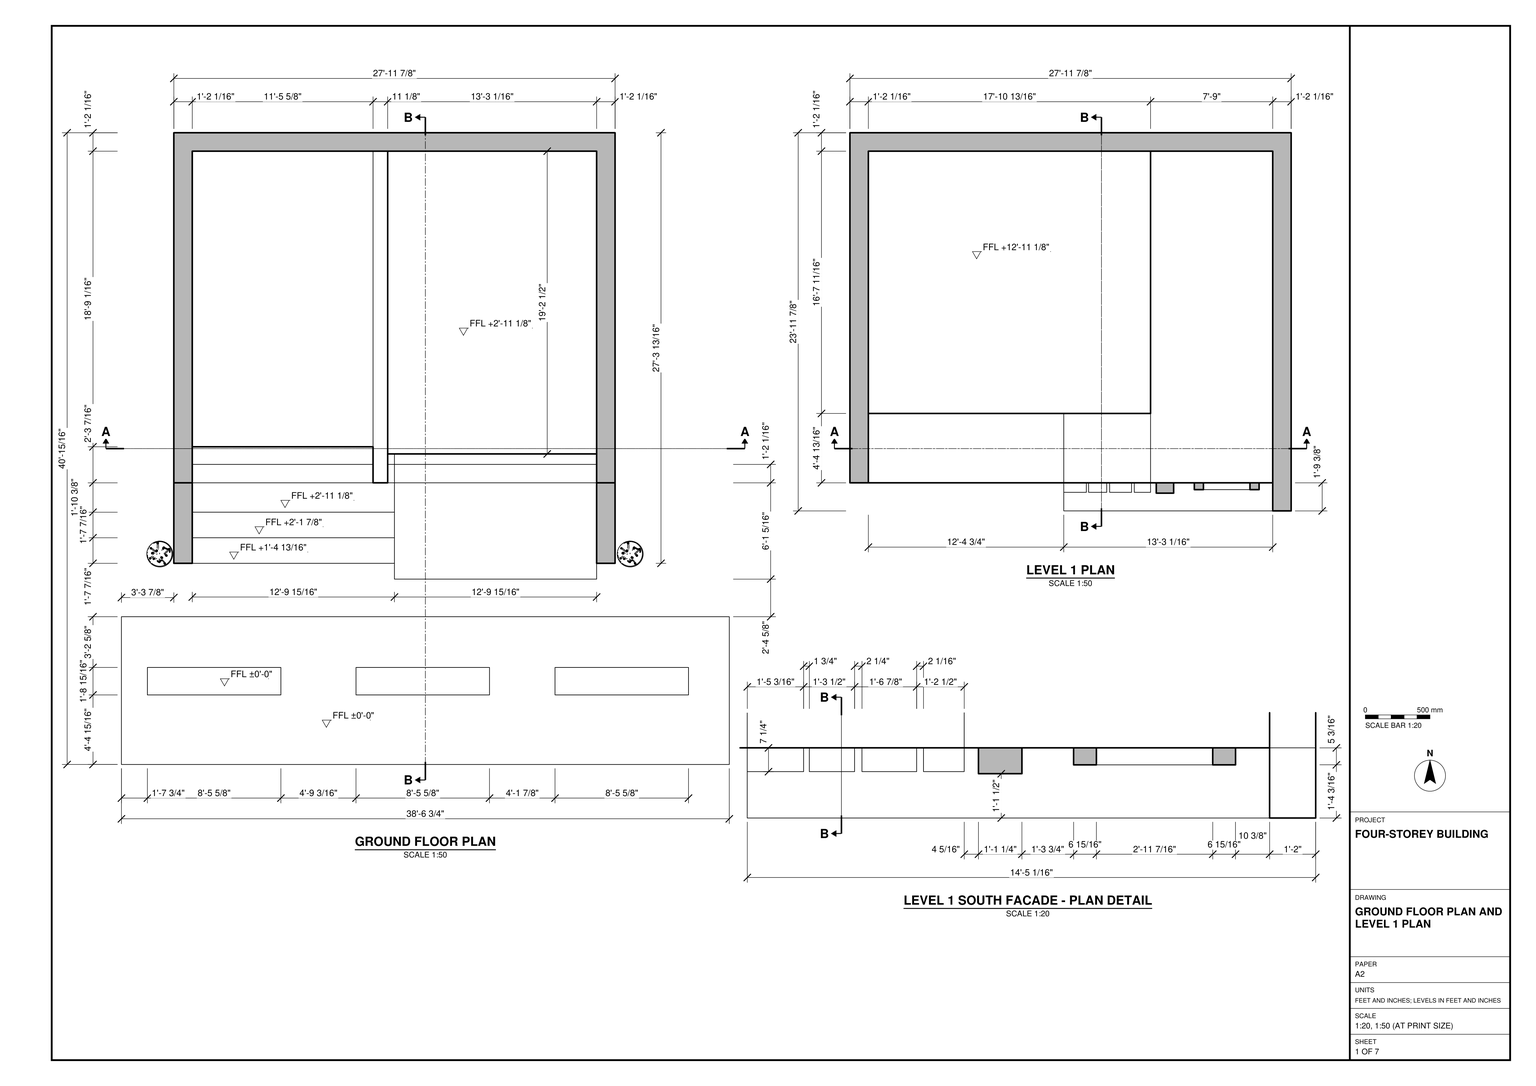
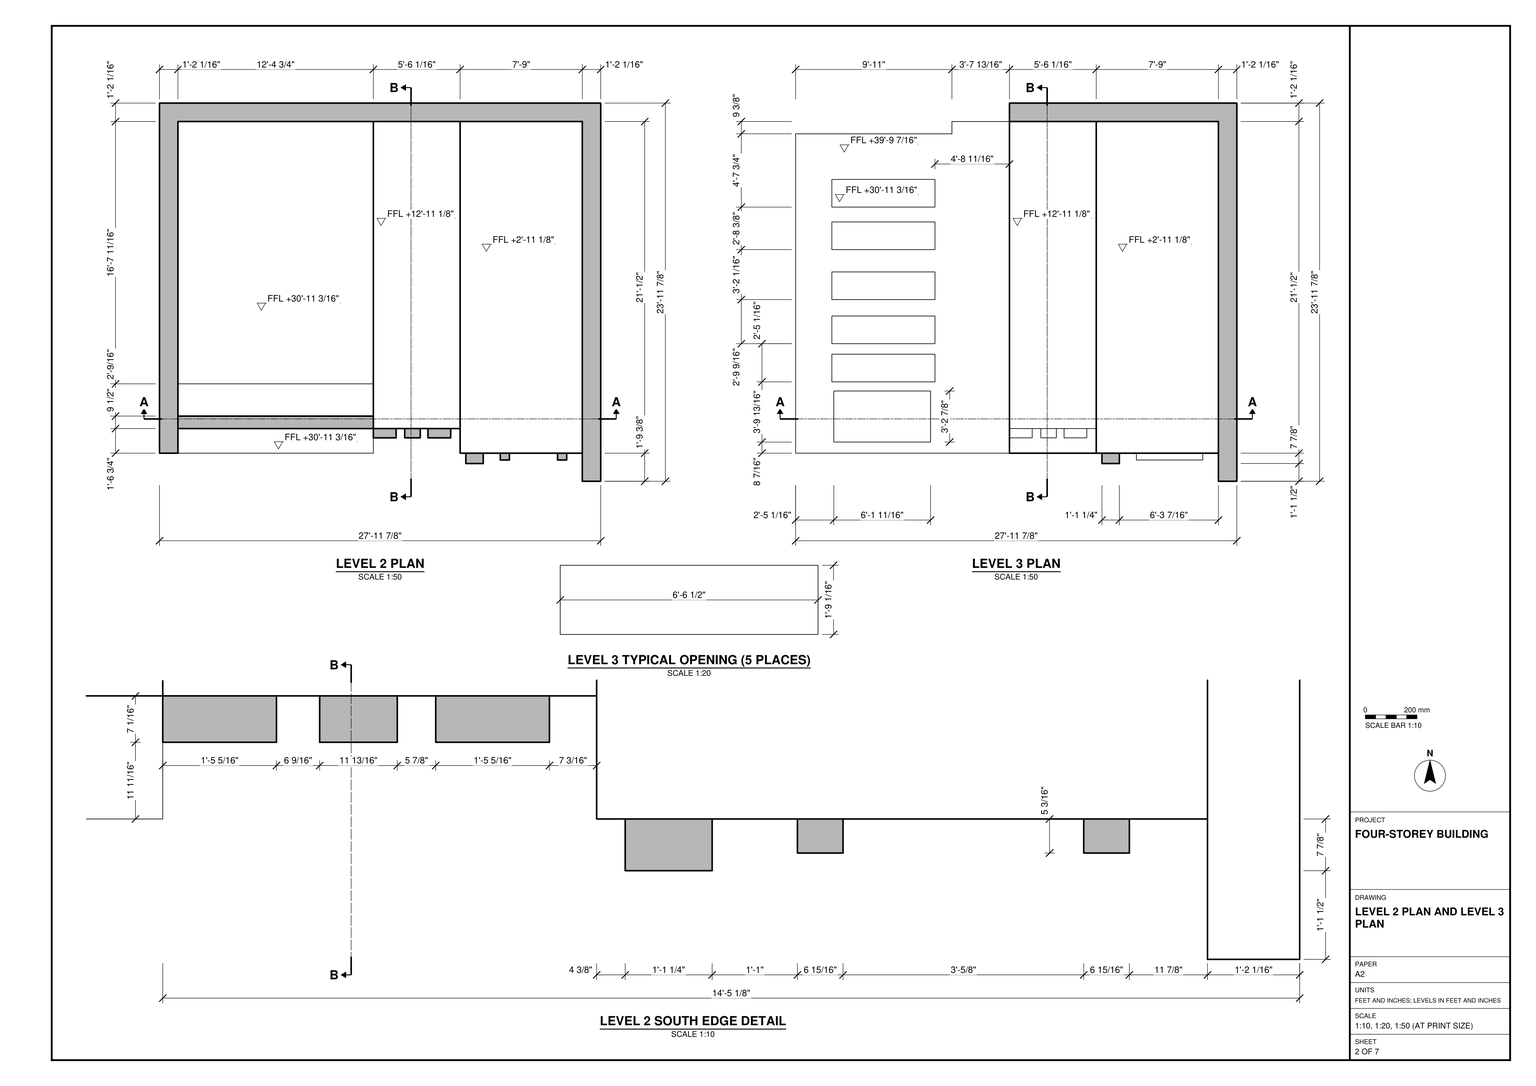
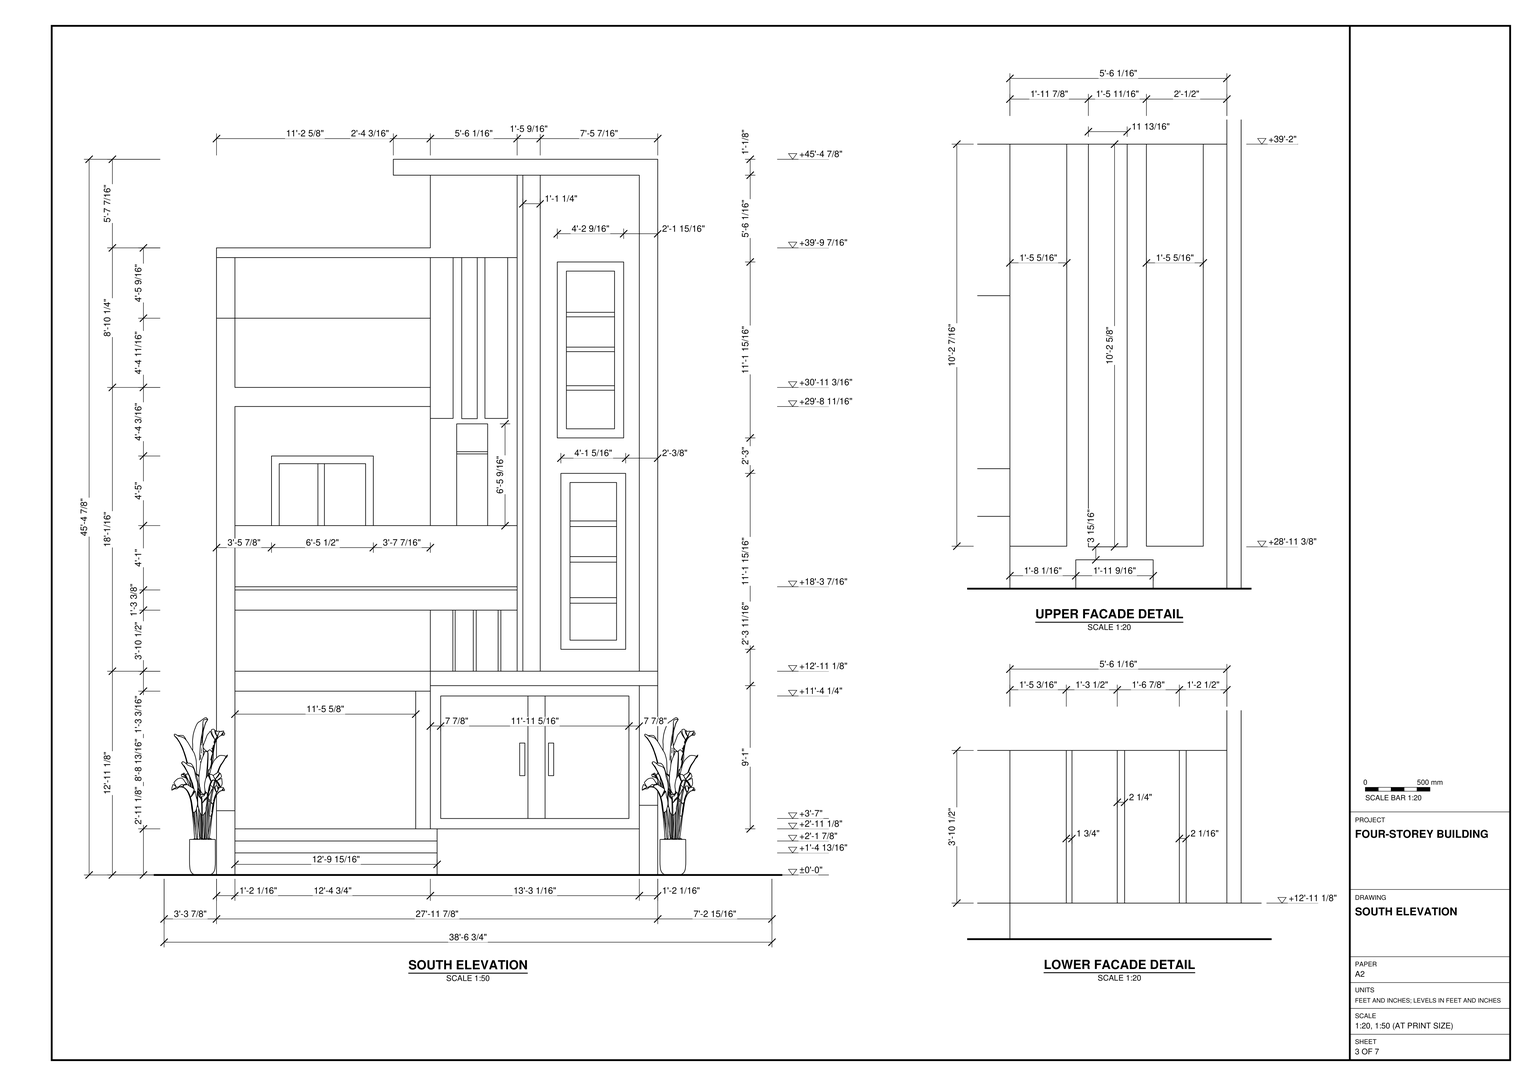
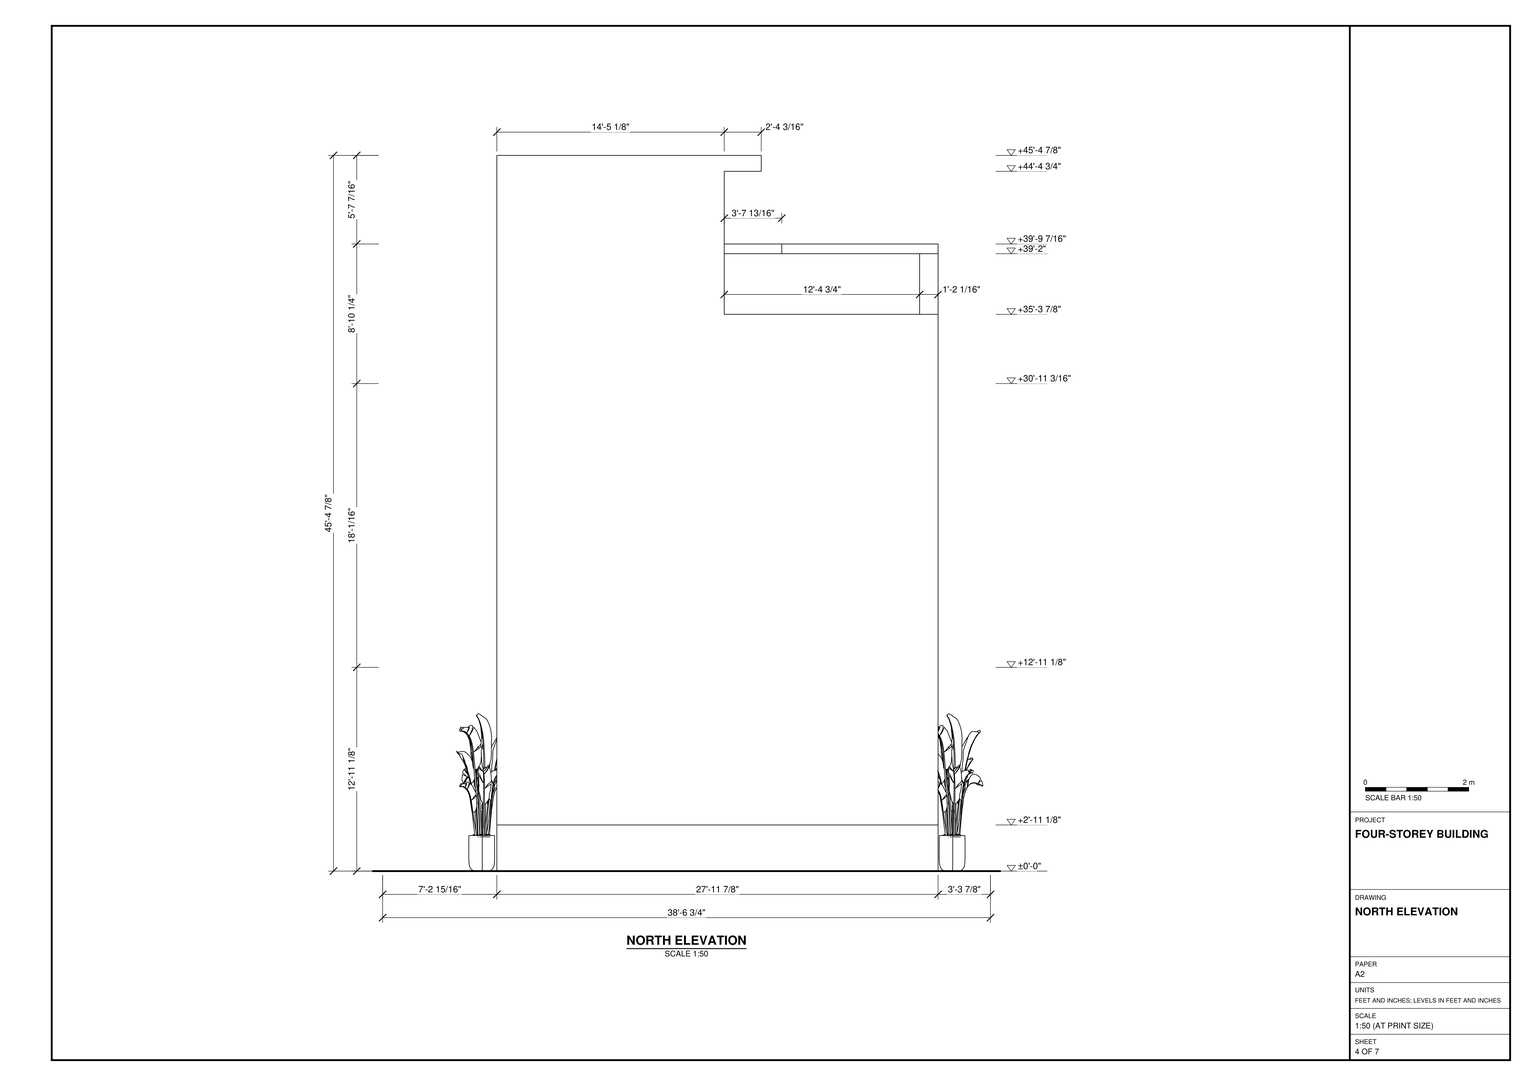
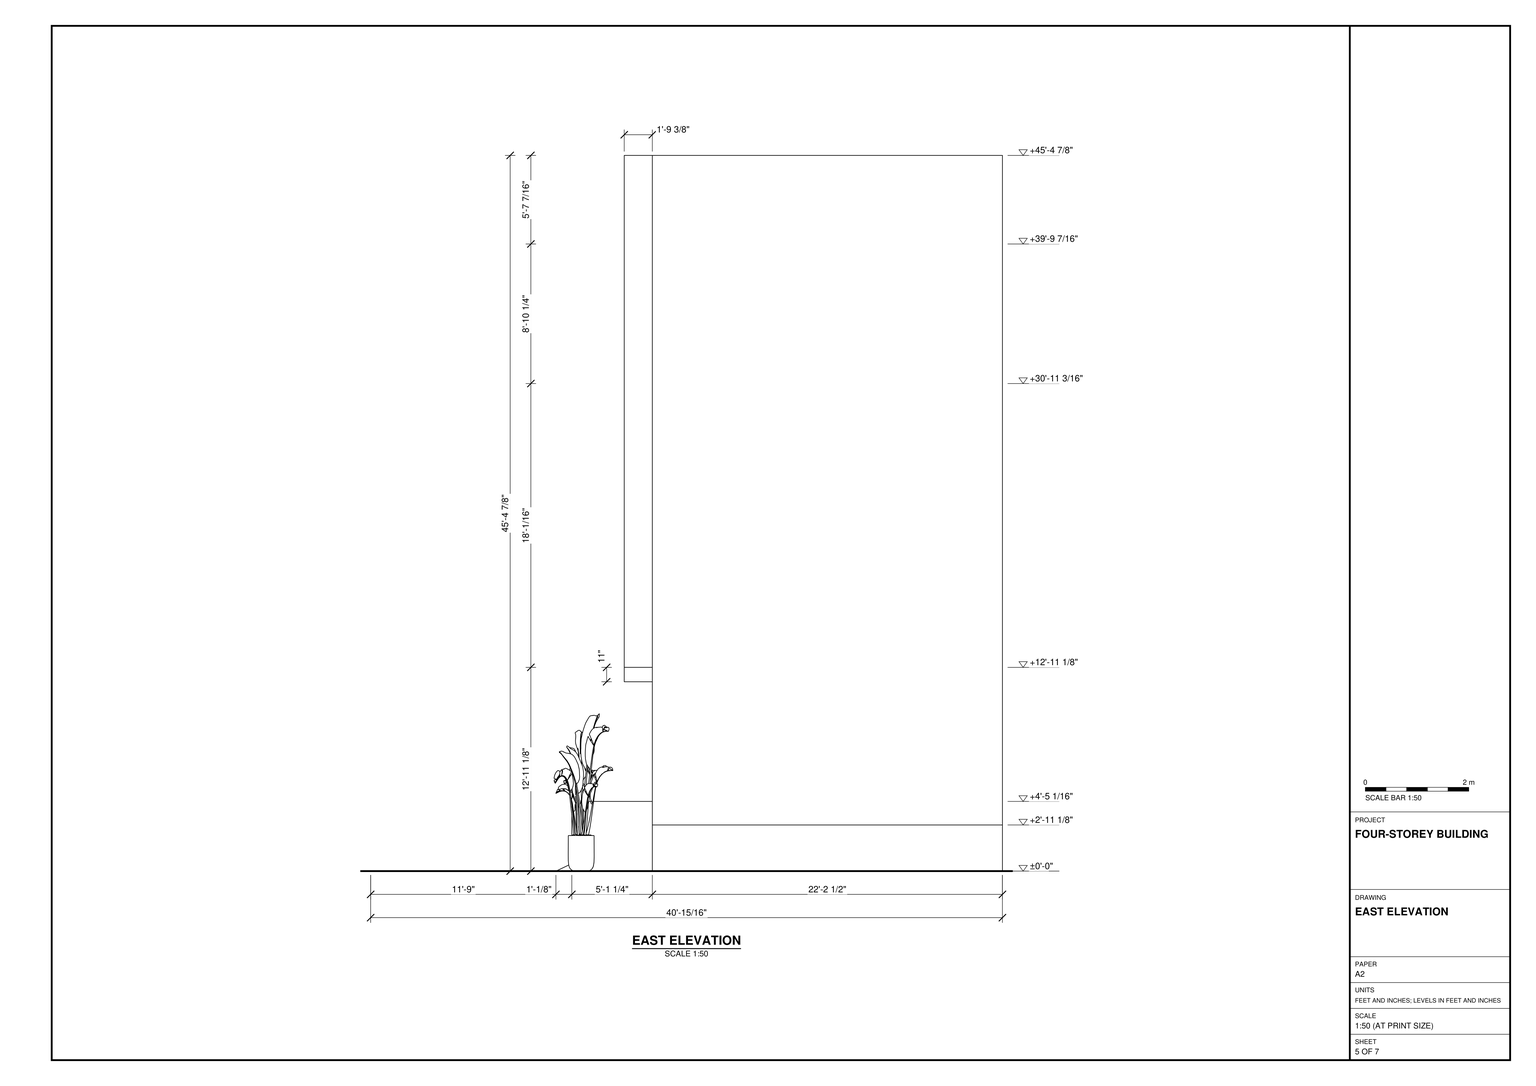
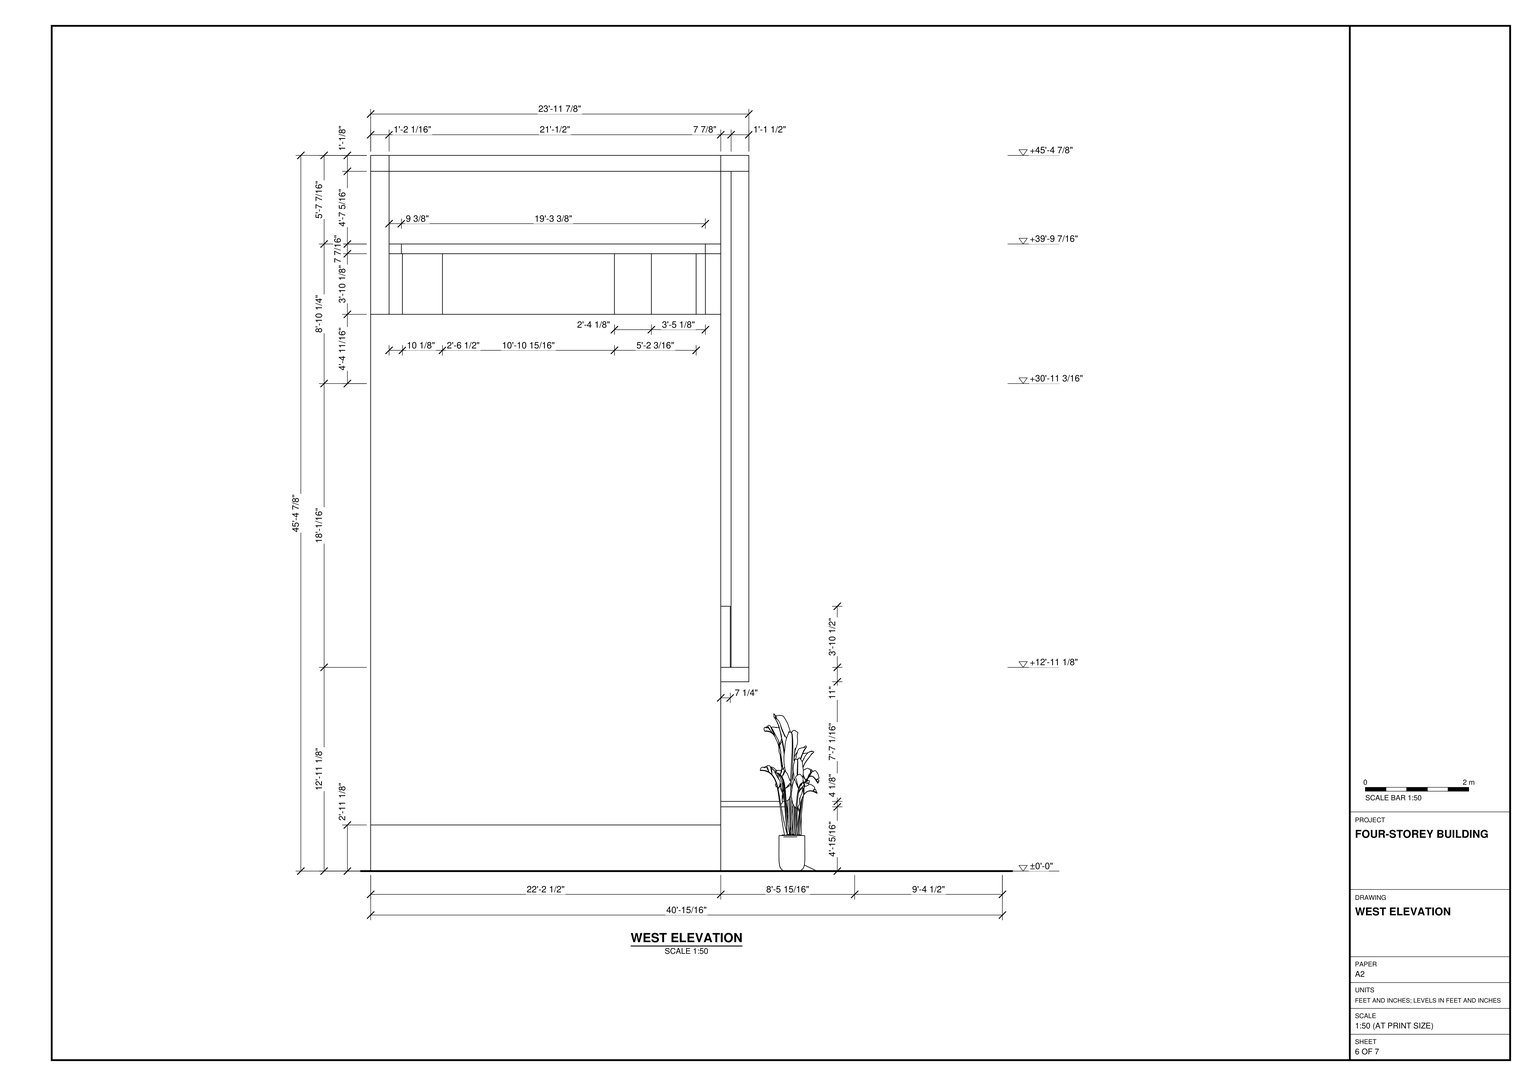
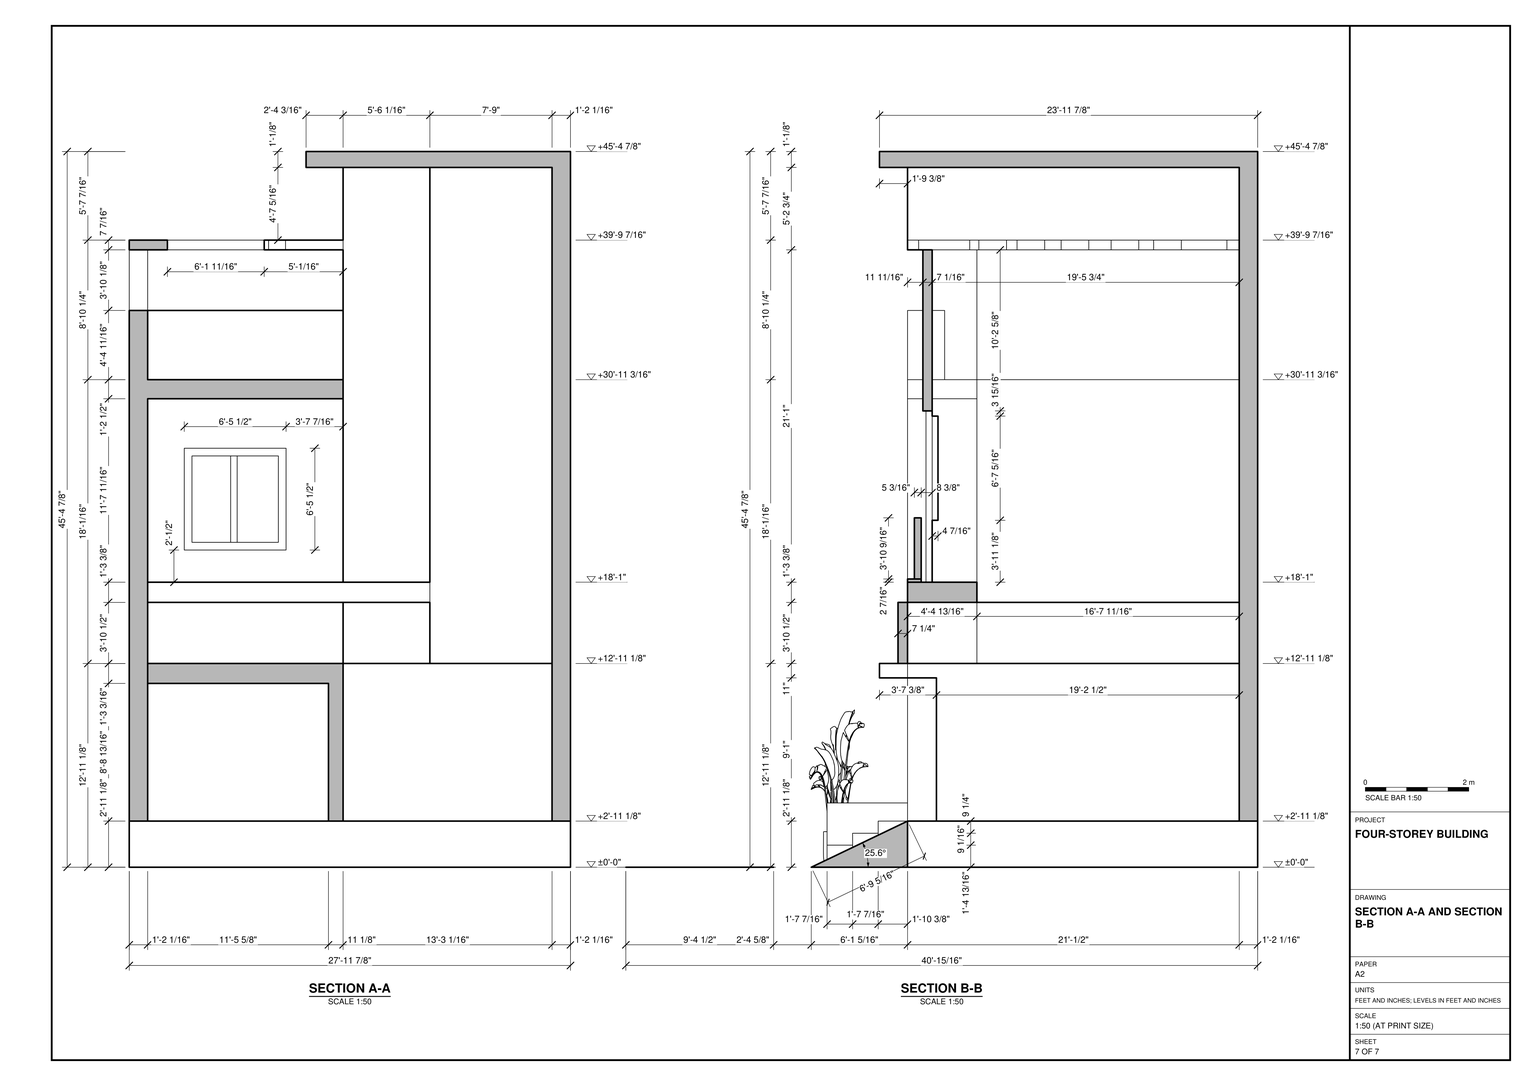
Build the four-storey building in SketchUp using task_files/diagram_01.pdf. Work in feet and inches, with X running east–west and Y running north–south. Including the forecourt and roof, the overall extents are 38'-6 3/4" along X, 40'-15/16" along Y and 45'-4 7/8" in height. Set the ground datum at ±0'-0", Level 1 at +12'-11 1/8", Level 2 at +30'-11 3/16" and Level 3 at +39'-9 7/16".

Distinguish the wider forecourt from the 27'-11 7/8" building body. Model the rear and side walls at their drawn thickness of 1'-2 1/16", the ground-floor dividing wall, the raised floor and the broad steps in the west entrance bay. Place the paired entrance doors in the east bay. Follow the slab outline at each level, retaining the areas open to the floors below. Cut the row of rectangular openings in the western Level 3 slab.

Use the south elevation and edge details to position the horizontal bands, narrow vertical projections, stacked window units and projecting flat roof. Include the planters flanking the entrance. Decor and loose items, including plants, may be suitable library components. Keep walls, slabs, roof and each furniture or joinery piece shown in separate groups or components, and use components for repeated parts. Save one SketchUp model as output_files/four_storey_building_with_its_stepped_south_facade.skp.

# SketchUp Ruby script. Lengths in inches.
U = 1.inch
M = Sketchup.active_model
def pt(a) = Geom::Point3d.new(a.map { |v| v * U })
def face(e, loops, mat)
  f = e.add_face(loops[0].map { |a| pt(a) })
  loops[1..].each { |l| e.add_face(l.map { |a| pt(a) }).erase! }
  f.material = f.back_material = mat if mat
  f
end
# faces: each face lists its corners as indices into pts; further lists are holes
def faces(e, pts, list, mat = nil) = list.each { |f| face(e, (f[0].is_a?(Array) ? f : [f]).map { |l| l.map { |i| pts[i] } }, mat) }
# xy, xz, yz: faces in a plane at the given z, y or x. An outline is a flat list of corners, or four numbers for a rectangle; further outlines are holes
def ring(l) = l.size == 4 ? [[l[0], l[1]], [l[2], l[1]], [l[2], l[3]], [l[0], l[3]]] : l.each_slice(2).to_a
def flat(e, list, mat, &to3) = list.each { |f| face(e, (f[0].is_a?(Array) ? f : [f]).map { |l| ring(l).map { |u, v| to3.(u, v) } }, mat) }
def xy(e, z, list, mat = nil) = flat(e, list, mat) { |x, y| [x, y, z] }
def xz(e, y, list, mat = nil) = flat(e, list, mat) { |x, z| [x, y, z] }
def yz(e, x, list, mat = nil) = flat(e, list, mat) { |y, z| [x, y, z] }
def lines(e, pts, list) = list.each { |a, b| e.add_line(pt(pts[a]), pt(pts[b])) }
# prism: a flat outline (further loops are holes) pulled along v
def prism(e, loops, v, mat = nil)
  f = face(e, loops, mat); d = Geom::Vector3d.new(v.map { |x| x * U })
  f.pushpull(f.normal.samedirection?(d) ? d.length : -d.length)
end
def box(e, o, s, mat = nil) = prism(e, [[o, [o[0] + s[0], o[1], o[2]], [o[0] + s[0], o[1] + s[1], o[2]], [o[0], o[1] + s[1], o[2]]]], [0, 0, s[2]], mat)
def at(x, y, z, deg = 0) = Geom::Transformation.translation(pt([x, y, z])) * Geom::Transformation.rotation(ORIGIN, Z_AXIS, deg.degrees)
def axes(o, x, y, z) = Geom::Transformation.new([*x, 0, *y, 0, *z, 0, *pt(o).to_a, 1])
def part(name) = M.definitions.add(name)
# library, detail: a bought-in or finely detailed component or shape, given as its bounding box
def library(name, o, s) = part(name).tap { |d| box(d.entities, o, s) }
def detail(e, o, s) = box(e.add_group.entities, o, s)
def put(e, d, t, mat = nil) = e.add_instance(d, t).tap { |i| i.material = mat if mat }
def group(e, t, mat = nil) = e.add_group.tap { |g| g.transformation = t; g.material = mat if mat }.entities
root = M.entities
M.materials.add("[Asphalt New]").color = [67, 60, 62]
M.materials.add("[Blinds Roman Hobbled Blue]").color = [49, 50, 53]
M.materials.add("[Blinds Vertical Pattern]").color = [232, 232, 234]
M.materials.add("[Blinds Vertical Pattern]1").color = [247, 247, 249]
M.materials.add("[Color C08]").color = [79, 39, 0]
M.materials.add("[Color C08]1").color = [102, 51, 0]
M.materials.add("[Color M00]").color = [255, 255, 255]
M.materials.add("[Color M06]").color = [86, 86, 86]
M.materials.add("[Formica Beige]").color = [211, 187, 149]
M.materials.add("[Formica Laminate Dark]").color = [50, 53, 60]
M.materials.add("[Formica Laminate Light]").color = [213, 189, 164]
M.materials.add("[Formica Speckled Grey]").color = [94, 105, 111]
M.materials.add("[Sandstone]").color = [118, 81, 52]
M.materials.add("[Terrazzo Tile Light]").color = [219, 217, 210]
M.materials.add("[Translucent Glass Gray]").color = [128, 128, 128]
M.materials["[Translucent Glass Gray]"].alpha = 0.5
M.materials.add("[Translucent Glass Safety]").color = [213, 245, 255]
M.materials["[Translucent Glass Safety]"].alpha = 0.19
M.materials.add("[Translucent Glass Safety]1").color = [204, 235, 244]
M.materials["[Translucent Glass Safety]1"].alpha = 0.5
M.materials.add("[Wood Cherry Original]").color = [152, 86, 42]
M.materials.add("[Wood Floor Light]").color = [204, 176, 127]
M.materials.add("[Wood Floor Parquet]").color = [145, 89, 39]
M.materials.add("[Wood Floor]").color = [155, 105, 61]
M.materials.add("[Wood Veneer 01]").color = [63, 37, 19]
M.materials.add("[Wood Veneer 01]1").color = [120, 70, 37]
M.materials.add("[Wood Veneer 02]").color = [190, 128, 91]
c1 = library("chau cay",[-24.34,-109.24,0],[56.46,62.58,79.69])
xy(root,0,[[207.84,141.12,361.75,153.16],[39.89,153.16,39.89,480.95,375.78,480.95,375.78,214.43,53.92,214.43,53.92,153.16],[53.92,153.16,207.84,172.61],[207.84,153.16,361.75,214.43],[361.75,153.16,375.78,214.43],
  [53.92,172.61,207.84,192.07],[53.92,192.07,207.84,214.43]])
xy(root,0,[[19.76,52.95,121.39,73.89],[178.57,52.95,280.2,73.89],[330.07,52.95,431.7,73.89]],"[Color M00]")
xy(root,0,[[[0,0,462.75,112.5],[19.76,52.95,121.39,73.89],[178.57,52.95,280.2,73.89],[330.07,52.95,431.7,73.89]]],"[Color M06]")
xy(root,16.8125,[[53.92,153.16,207.84,172.61]],"[Terrazzo Tile Light]")
xy(root,25.875,[[53.92,172.61,207.84,192.07]],"[Terrazzo Tile Light]")
xy(root,35.125,[[39.89,214.43,39.89,480.95,375.78,480.95,375.78,214.43,361.75,214.43,361.75,466.92,53.92,466.92,53.92,214.43],[191.55,214.43,202.6875,466.92],[202.6875,236.43,361.75,466.92],[53.92,241.87,191.55,466.92]])
xy(root,35.125,[[53.92,192.07,207.84,214.43],[53.92,214.43,191.55,228.46],[202.6875,214.43,207.84,228.46],[207.84,214.43,361.75,228.46],[53.92,228.46,191.55,241.87],
  [202.6875,228.46,207.84,236.43],[207.84,228.46,361.75,236.43]],"[Terrazzo Tile Light]")
xy(root,48.9375,[[39.89,153.16,53.92,214.43]],"[Terrazzo Tile Light]")
xy(root,53.0625,[[361.75,153.16,375.78,214.43]],"[Terrazzo Tile Light]")
xy(root,139.93,[[53.92,214.43,191.55,241.87]],"[Asphalt New]")
xy(root,144.15,[[202.6875,193.05,202.6875,236.43,361.75,236.43,361.75,214.43,375.78,214.43,375.78,193.05]],"[Blinds Vertical Pattern]")
xy(root,155.125,[[361.75,193.05,375.78,214.43],[273.09,206.55,286.33,214.43],[202.6875,207.18,219.85,214.43],[221.59,207.18,235.375,214.43],[237.62,207.18,254.28,214.43],
  [256.36,207.18,268.75,214.43],[202.6875,214.43,268.75,466.92],[268.75,214.43,361.75,466.92],[53.92,267.23,191.55,466.92],[191.55,267.23,202.6875,466.92]])
xy(root,155.125,[[202.6875,193.05,361.75,193.05,361.75,214.43,286.33,214.43,286.33,206.55,273.09,206.55,273.09,214.43,268.75,214.43,268.75,207.18,256.36,207.18,256.36,214.43,254.28,214.43,254.28,207.18,237.62,207.18,237.62,214.43,235.375,214.43,235.375,207.18,221.59,207.18,221.59,214.43,219.85,214.43,219.85,207.18,202.6875,207.18],[53.92,214.43,191.55,267.23],[191.55,214.43,202.6875,267.23]],"[Blinds Vertical Pattern]")
xy(root,171.81,[[302.07,209.24,351.38,214.43]],"[Color C08]")
xy(root,178.76,[[309.01,209.24,344.43,214.43]],"[Color C08]")
xy(root,201.625,[[202.6875,214.43,268.75,267.23],[53.92,267.23,268.75,466.92]])
xy(root,201.625,[[53.92,214.43,202.6875,267.23]],"[Wood Cherry Original]")
xy(root,201.625,[[202.6875,207.18,219.85,214.43],[221.59,207.18,235.375,214.43],[237.62,207.18,254.28,214.43],[256.36,207.18,268.75,214.43]],"[Wood Veneer 02]")
xy(root,216.99,[[53.92,214.43,268.75,224.81],[53.92,224.81,202.6875,267.23],[202.6875,224.81,268.75,233.17],[202.6875,233.17,268.75,267.23]])
xy(root,219.43,[[53.92,214.43,268.75,219.62],[53.92,219.62,268.75,224.81]])
xy(root,264.13,[[222.75,233.17,246.31,237.61]],"[Formica Laminate Light]")
xy(root,265.99,[[53.92,219.62,268.75,224.81]])
xy(root,298.8,[[309.01,209.24,344.43,214.43]],"[Color C08]")
xy(root,305.75,[[302.07,209.24,351.38,214.43]],"[Wood Veneer 01]1")
xy(root,332.75,[[299.32,209.24,349.86,214.43]],"[Color C08]")
xy(root,339.69,[[306.26,209.24,342.91,214.43]],"[Color C08]")
xy(root,343.44,[[222.75,233.17,246.31,237.61]],"[Formica Laminate Light]")
xy(root,347.39,[[226.58,226.11,238.39,233.17]],"[Wood Veneer 02]")
xy(root,347.58,[[202.6875,226.11,220,233.17],[244.25,226.11,261.5625,233.17]],"[Wood Veneer 02]")
xy(root,356.67,[[53.92,214.43,202.6875,228.46]],"[Blinds Vertical Pattern]")
xy(root,356.67,[[53.92,228.46,202.6875,267.23]],"[Wood Cherry Original]")
xy(root,371.1875,[[53.92,214.43,202.6875,233.17],[53.92,233.17,202.6875,242.66],[53.92,242.66,202.6875,267.23],[53.92,267.23,202.6875,466.92]])
xy(root,423.875,[[39.89,267.23,53.92,295.36],[39.89,426.29,53.92,456.77]])
xy(root,423.875,[[39.89,214.43,53.92,267.23],[53.92,233.17,202.6875,242.66],[39.89,295.36,53.92,426.29],[39.89,456.77,53.92,456.77,53.92,466.92,202.6875,466.92,202.6875,480.95,39.89,480.95]],"[Blinds Vertical Pattern]")
xy(root,459.74,[[306.26,209.24,342.91,214.43]],"[Sandstone]")
xy(root,466.68,[[299.32,209.24,349.86,214.43]],"[Color C08]")
xy(root,470.02,[[202.6875,226.11,220,233.17],[226.58,226.11,238.39,233.17],[244.25,226.11,261.5625,233.17]])
xy(root,470.02,[[[39.89,214.43,39.89,267.23,53.92,267.23,53.92,295.36,39.89,295.36,39.89,426.29,53.92,426.29,53.92,456.77,39.89,456.77,39.89,457.55,158.875,457.55,158.875,466.92,202.6875,466.92,202.6875,226.11,220,226.11,220,233.17,226.58,233.17,226.58,226.11,238.39,226.11,238.39,233.17,244.25,233.17,244.25,226.11,261.5625,226.11,261.5625,233.17,268.75,233.17,268.75,214.43],[164.65,234.83,193.97,419.64],[68.95,222.9,142.63,261.77],[67.48,297.78,145.98,318.84],[67.48,331.34,145.98,352.41],[67.48,268.72,145.98,289.78],[67.48,369.41,145.98,390.47],[67.48,401.78,145.98,422.84]]],"[Blinds Vertical Pattern]")
xy(root,470.02,[[168.46,238.63,190.16,415.84]],"[Color C08]1")
xy(root,470.02,[[[164.65,234.83,193.97,419.64],[168.46,238.63,190.16,415.84]]],"[Formica Beige]")
xy(root,477.4375,[[[39.89,214.43,202.6875,214.43,202.6875,466.92,158.875,466.92,158.875,457.55,39.89,457.55],[68.95,222.9,142.63,261.77],[67.48,331.34,145.98,352.41],[67.48,297.78,145.98,318.84],[67.48,369.41,145.98,390.47],[67.48,268.72,145.98,289.78],[67.48,401.78,145.98,422.84]]],"[Blinds Vertical Pattern]")
xy(root,532.75,[[273.09,206.55,286.33,214.43],[202.6875,214.43,268.75,228.46],[268.75,214.43,361.75,228.46],[202.6875,228.46,268.75,466.92],[268.75,228.46,361.75,466.92],
  [174.5,466.92,202.6875,480.95]])
xy(root,532.75,[[174.5,193.05,174.5,466.92,202.6875,466.92,202.6875,214.43,273.09,214.43,273.09,206.55,286.33,206.55,286.33,214.43,361.75,214.43,361.75,193.05]],"[Blinds Vertical Pattern]")
xy(root,544.875,[[174.5,193.05,375.78,214.43],[174.5,214.43,375.78,480.95]],"[Blinds Vertical Pattern]1")
xz(root,153.16,[[39.89,0,53.92,48.9375],[53.92,0,207.84,16.8125],[361.75,0,375.78,53.0625]],"[Terrazzo Tile Light]")
xz(root,172.61,[[53.92,0,207.84,16.8125]])
xz(root,172.61,[[53.92,16.8125,207.84,25.875]],"[Terrazzo Tile Light]")
xz(root,192.07,[[53.92,0,207.84,25.875]])
xz(root,192.07,[[53.92,25.875,207.84,35.125]],"[Terrazzo Tile Light]")
xz(root,193.05,[[202.6875,144.15,375.78,155.125],[361.75,155.125,375.78,155.125,375.78,544.875,174.5,544.875,174.5,532.75,361.75,532.75]],"[Blinds Vertical Pattern]")
xz(root,206.55,[[273.09,155.125,286.33,532.75]],"[Wood Veneer 02]")
xz(root,207.18,[[202.6875,155.125,219.85,201.625],[221.59,155.125,235.375,201.625],[237.62,155.125,254.28,201.625],[256.36,155.125,268.75,201.625]],"[Wood Veneer 02]")
xz(root,209.24,[[[302.07,171.81,351.38,305.75],[309.01,178.76,344.43,298.8]],[[299.32,332.75,349.86,466.68],[306.26,339.69,342.91,459.74]]],"[Color C08]")
xz(root,214.43,[[53.92,0,207.84,35.125],[207.84,0,361.75,35.125],[361.75,0,375.78,35.125],[39.89,35.125,53.92,48.9375],[361.75,35.125,375.78,53.0625],
  [361.75,144.15,375.78,155.125],[202.6875,155.125,219.85,201.625],[219.85,155.125,221.59,201.625],[221.59,155.125,235.375,201.625],[235.375,155.125,237.62,201.625],
  [237.62,155.125,254.28,201.625],[254.28,155.125,256.36,201.625],[256.36,155.125,268.75,201.625],[273.09,155.125,286.33,532.75],[[302.07,171.81,351.38,305.75],[309.01,178.76,344.43,298.8]],
  [53.92,216.99,268.75,219.43],[[299.32,332.75,349.86,466.68],[306.26,339.69,342.91,459.74]]])
xz(root,214.43,[[53.92,139.93,202.6875,155.125]],"[Asphalt New]")
xz(root,214.43,[[191.55,35.125,202.6875,139.93],[361.75,53.0625,375.78,144.15],[268.75,155.125,273.09,532.75],[[286.33,155.125,361.75,532.75],[299.32,332.75,349.86,466.68],[302.07,171.81,351.38,305.75]],[39.89,470.02,268.75,470.02,268.75,532.75,202.6875,532.75,202.6875,477.4375,39.89,477.4375]],"[Blinds Vertical Pattern]")
xz(root,214.43,[[39.89,48.9375,53.92,48.9375,53.92,356.67,202.6875,356.67,202.6875,371.1875,53.92,371.1875,53.92,423.875,39.89,423.875],[53.92,201.625,268.75,216.99]],"[Blinds Vertical Pattern]1")
xz(root,214.43,[[309.01,178.76,344.43,206.89],[309.01,206.89,344.43,211.14],[309.01,211.14,344.43,238.14],[309.01,238.14,344.43,242.39],[309.01,242.39,344.43,265.27],
  [309.01,265.27,344.43,269.52],[309.01,269.52,344.43,298.8],[306.26,339.69,342.91,369.05],[306.26,369.05,342.91,372.5],[306.26,372.5,342.91,398.42],
  [306.26,398.42,342.91,401.86],[306.26,401.86,342.91,424.92],[306.26,424.92,342.91,428.36],[306.26,428.36,342.91,459.74]],"[Sandstone]")
xz(root,219.62,[[53.92,219.43,268.75,265.99]],"[Translucent Glass Safety]")
xz(root,222.9,[[68.95,470.02,142.63,477.4375]],"[Blinds Vertical Pattern]")
xz(root,224.81,[[53.92,216.99,202.6875,219.43],[202.6875,216.99,268.75,219.43]])
xz(root,224.81,[[53.92,219.43,202.6875,265.99],[202.6875,219.43,268.75,265.99]],"[Translucent Glass Safety]")
xz(root,226.11,[[226.58,347.39,238.39,470.02],[202.6875,347.58,220,470.02],[244.25,347.58,261.5625,470.02]],"[Wood Veneer 02]")
xz(root,233.17,[[226.58,347.39,238.39,470.02],[202.6875,347.58,220,470.02],[244.25,347.58,261.5625,470.02]])
xz(root,233.17,[[[202.6875,216.99,204.91,216.99,204.91,262.18,217.35,262.18,217.35,216.99,221.29,216.99,221.29,262.18,233.72,262.18,233.72,216.99,238.1,216.99,238.1,262.18,250.54,262.18,250.54,216.99,256.3125,216.99,256.3125,262.18,268.75,262.18,268.75,470.02,261.5625,470.02,261.5625,347.58,244.25,347.58,244.25,470.02,238.39,470.02,238.39,347.39,226.58,347.39,226.58,470.02,220,470.02,220,347.58,202.6875,347.58],[222.75,264.13,246.31,343.44]]],"[Blinds Vertical Pattern]1")
xz(root,233.17,[[53.92,371.1875,202.6875,423.875]],"[Translucent Glass Safety]1")
xz(root,233.17,[[204.91,216.99,217.35,262.18],[221.29,216.99,233.72,262.18],[238.1,216.99,250.54,262.18],[256.3125,216.99,268.75,262.18]],"[Wood Floor Parquet]")
xz(root,236.43,[[[202.6875,35.125,361.75,144.15],[210.57,43.01,353.87,136.27]]],"[Blinds Vertical Pattern]")
xz(root,236.43,[[270.67,75.625,274.65,100.44],[292.61,75.625,296.59,100.44]],"[Formica Laminate Dark]")
xz(root,236.43,[[[210.57,43.01,277,136.27],[270.67,75.625,274.65,100.44]],[277,43.01,290.04,136.27],[[290.04,43.01,353.87,136.27],[292.61,75.625,296.59,100.44]]],"[Wood Veneer 01]")
xz(root,237.61,[[222.75,320.57,246.31,322.24]],"[Formica Speckled Grey]")
xz(root,237.61,[[222.75,322.24,246.31,343.44]],"[Wood Floor Light]")
xz(root,237.61,[[222.75,264.13,246.31,320.57]],"[Wood Floor]")
xz(root,241.87,[[53.92,35.125,191.55,139.93]],"[Blinds Roman Hobbled Blue]")
xz(root,242.66,[[53.92,371.1875,202.6875,423.875]],"[Translucent Glass Safety]1")
xz(root,261.77,[[68.95,470.02,142.63,477.4375]],"[Blinds Vertical Pattern]")
xz(root,267.23,[[53.92,201.625,268.75,216.99],[53.92,356.67,202.6875,371.1875]])
xz(root,267.23,[[53.92,155.125,202.6875,201.625],[[53.92,216.99,202.6875,356.67],[81.78,241.48,159.28,318.98]],[39.89,423.875,53.92,470.02]],"[Blinds Vertical Pattern]")
xz(root,267.23,[[[81.78,241.48,159.28,318.98],[87.64,247.35,153.41,313.12]],[117.09,247.35,122.04,313.12]],"[Formica Laminate Dark]")
xz(root,267.23,[[87.64,247.35,117.09,313.12],[122.04,247.35,153.41,313.12]],"[Translucent Glass Gray]")
xz(root,268.72,[[67.48,470.02,145.98,477.4375]],"[Blinds Vertical Pattern]")
xz(root,289.78,[[67.48,470.02,145.98,477.4375]],"[Blinds Vertical Pattern]")
xz(root,295.36,[[39.89,423.875,53.92,470.02]],"[Blinds Vertical Pattern]")
xz(root,297.78,[[67.48,470.02,145.98,477.4375]],"[Blinds Vertical Pattern]")
xz(root,318.84,[[67.48,470.02,145.98,477.4375]],"[Blinds Vertical Pattern]")
xz(root,331.34,[[67.48,470.02,145.98,477.4375]],"[Blinds Vertical Pattern]")
xz(root,352.41,[[67.48,470.02,145.98,477.4375]],"[Blinds Vertical Pattern]")
xz(root,369.41,[[67.48,470.02,145.98,477.4375]],"[Blinds Vertical Pattern]")
xz(root,390.47,[[67.48,470.02,145.98,477.4375]],"[Blinds Vertical Pattern]")
xz(root,401.78,[[67.48,470.02,145.98,477.4375]],"[Blinds Vertical Pattern]")
xz(root,422.84,[[67.48,470.02,145.98,477.4375]],"[Blinds Vertical Pattern]")
xz(root,426.29,[[39.89,423.875,53.92,470.02]],"[Blinds Vertical Pattern]")
xz(root,456.77,[[39.89,423.875,53.92,470.02]],"[Blinds Vertical Pattern]")
xz(root,457.55,[[39.89,470.02,158.875,477.4375]],"[Blinds Vertical Pattern]")
xz(root,466.92,[[53.92,35.125,191.55,155.125],[191.55,35.125,202.6875,155.125],[202.6875,35.125,361.75,155.125],[53.92,155.125,268.75,201.625],[268.75,155.125,361.75,532.75],
  [53.92,201.625,53.92,371.1875,202.6875,371.1875,202.6875,532.75,268.75,532.75,268.75,201.625]])
xz(root,466.92,[[53.92,371.1875,202.6875,423.875],[158.875,470.02,202.6875,477.4375]],"[Blinds Vertical Pattern]")
xz(root,480.95,[[39.89,0,375.78,35.125]],"[Blinds Vertical Pattern]")
xz(root,480.95,[[39.89,35.125,39.89,423.875,202.6875,423.875,202.6875,532.75,174.5,532.75,174.5,544.875,375.78,544.875,375.78,35.125]],"[Blinds Vertical Pattern]1")
yz(root,39.89,[[214.43,0,480.95,35.125],[267.23,423.875,295.36,470.02],[426.29,423.875,456.77,470.02],[214.43,470.02,226.18,477.4375],[226.18,470.02,457.55,477.4375]],"[Blinds Vertical Pattern]")
yz(root,39.89,[[214.43,35.125,480.95,423.875]],"[Blinds Vertical Pattern]1")
yz(root,39.89,[[153.16,0,214.43,48.9375]],"[Terrazzo Tile Light]")
yz(root,53.92,[[153.16,0,172.61,16.8125],[172.61,0,192.07,25.875],[192.07,0,214.43,35.125],[241.87,35.125,241.87,139.93,228.46,139.93,228.46,155.125,466.92,155.125,466.92,35.125],[214.43,139.93,228.46,155.125],
  [267.23,155.125,466.92,201.625],[214.43,201.625,228.46,216.99],[228.46,201.625,267.23,216.99],[267.23,201.625,466.92,371.1875],[214.43,216.99,224.81,219.43],
  [219.62,219.43,224.81,265.99],[214.43,371.1875,233.17,423.875],[233.17,371.1875,242.66,423.875],[242.66,371.1875,267.23,423.875]])
yz(root,53.92,[[214.43,35.125,228.46,139.93],[228.46,35.125,241.87,139.93],[214.43,155.125,228.46,201.625],[228.46,155.125,267.23,201.625],[224.81,216.99,228.46,216.99,228.46,356.67,214.43,356.67,214.43,219.43,219.62,219.43,219.62,265.99,224.81,265.99],
  [228.46,216.99,267.23,356.67],[267.23,371.1875,466.92,423.875],[267.23,423.875,295.36,470.02],[426.29,423.875,456.77,470.02]],"[Blinds Vertical Pattern]")
yz(root,53.92,[[153.16,16.8125,172.61,16.8125,172.61,25.875,192.07,25.875,192.07,35.125,214.43,35.125,214.43,48.9375,153.16,48.9375]],"[Terrazzo Tile Light]")
yz(root,67.48,[[297.78,470.02,318.84,477.4375],[331.34,470.02,352.41,477.4375],[369.41,470.02,390.47,477.4375],[401.78,470.02,422.84,477.4375]])
yz(root,67.48,[[268.72,470.02,289.78,477.4375]],"[Blinds Vertical Pattern]")
yz(root,68.95,[[222.9,470.02,261.77,477.4375]],"[Blinds Vertical Pattern]")
yz(root,142.63,[[222.9,470.02,261.77,477.4375]],"[Blinds Vertical Pattern]")
yz(root,145.98,[[268.72,470.02,289.78,477.4375],[297.78,470.02,318.84,477.4375],[331.34,470.02,352.41,477.4375],[369.41,470.02,390.47,477.4375],[401.78,470.02,422.84,477.4375]],"[Blinds Vertical Pattern]")
yz(root,158.875,[[457.55,470.02,466.92,477.4375]],"[Blinds Vertical Pattern]")
yz(root,174.5,[[193.05,532.75,214.43,544.875],[214.43,532.75,466.92,544.875],[466.92,532.75,480.95,544.875]],"[Blinds Vertical Pattern]")
yz(root,191.55,[[214.43,35.125,241.87,139.93]],"[Blinds Vertical Pattern]")
yz(root,202.6875,[[236.43,35.125,466.92,35.125,466.92,155.125,214.43,155.125,214.43,144.15,236.43,144.15],[193.05,144.15,214.43,155.125],[214.43,356.67,226.11,371.1875],[226.11,356.67,233.17,371.1875],[233.17,356.67,267.23,371.1875],
  [233.17,371.1875,242.66,423.875]])
yz(root,202.6875,[[214.43,35.125,236.43,144.15],[214.43,155.125,267.23,201.625],[233.17,216.99,267.23,356.67],[242.66,371.1875,242.66,423.875,233.17,423.875,233.17,470.02,267.23,470.02,267.23,371.1875],[267.23,371.1875,466.92,470.02],
  [466.92,423.875,480.95,532.75],[214.43,477.4375,466.92,532.75]],"[Blinds Vertical Pattern]")
yz(root,202.6875,[[207.18,155.125,214.43,201.625],[226.11,347.58,233.17,356.67],[226.11,371.1875,233.17,423.875],[226.11,423.875,233.17,470.02]],"[Wood Veneer 02]")
yz(root,207.84,[[153.16,0,153.16,5.77,172.61,15.09,172.61,0],[172.61,0,172.61,15.09,192.07,24.41,192.07,0],[192.07,0,192.07,24.41,214.43,35.125,214.43,0]])
yz(root,207.84,[[141.12,0,153.16,5.77,153.16,0],[153.16,5.77,172.61,15.09,172.61,16.8125,153.16,16.8125],[172.61,15.09,192.07,24.41,192.07,25.875,172.61,25.875],[192.07,24.41,214.43,35.125,192.07,35.125]],"[Terrazzo Tile Light]")
yz(root,219.85,[[207.18,155.125,214.43,201.625]],"[Wood Veneer 02]")
yz(root,220,[[226.11,347.58,233.17,470.02]],"[Wood Veneer 02]")
yz(root,221.59,[[207.18,155.125,214.43,201.625]],"[Wood Veneer 02]")
yz(root,222.75,[[233.17,264.13,237.61,343.44]],"[Formica Laminate Light]")
yz(root,226.58,[[226.11,347.39,233.17,470.02]],"[Wood Veneer 02]")
yz(root,235.375,[[207.18,155.125,214.43,201.625]],"[Wood Veneer 02]")
yz(root,237.62,[[207.18,155.125,214.43,201.625]],"[Wood Veneer 02]")
yz(root,238.39,[[226.11,347.39,233.17,470.02]],"[Wood Veneer 02]")
yz(root,244.25,[[226.11,347.58,233.17,356.67],[226.11,356.67,233.17,371.1875],[226.11,371.1875,233.17,423.875],[226.11,423.875,233.17,470.02]],"[Wood Veneer 02]")
yz(root,246.31,[[233.17,264.13,237.61,343.44]],"[Formica Laminate Light]")
yz(root,254.28,[[207.18,155.125,214.43,201.625]],"[Wood Veneer 02]")
yz(root,256.36,[[207.18,155.125,214.43,201.625]],"[Wood Veneer 02]")
yz(root,261.5625,[[226.11,347.58,233.17,470.02]],"[Wood Veneer 02]")
yz(root,268.75,[[214.43,155.125,466.92,201.625],[267.23,201.625,466.92,201.625,466.92,532.75,214.43,532.75,214.43,470.02,233.17,470.02,233.17,216.99,267.23,216.99],[214.43,216.99,224.81,219.43],[219.62,219.43,224.81,265.99]])
yz(root,268.75,[[224.81,216.99,224.81,265.99,219.62,265.99,219.62,219.43,214.43,219.43,214.43,470.02,233.17,470.02,233.17,216.99]],"[Blinds Vertical Pattern]")
yz(root,268.75,[[207.18,155.125,214.43,201.625]],"[Wood Veneer 02]")
yz(root,273.09,[[206.55,155.125,214.43,532.75]],"[Wood Veneer 02]")
yz(root,286.33,[[206.55,155.125,214.43,532.75]],"[Wood Veneer 02]")
yz(root,299.32,[[209.24,332.75,214.43,466.68]],"[Color C08]")
yz(root,302.07,[[209.24,171.81,214.43,305.75]],"[Color C08]")
yz(root,306.26,[[209.24,339.69,214.43,459.74]],"[Color C08]")
yz(root,309.01,[[209.24,178.76,214.43,206.89],[209.24,206.89,214.43,211.14],[209.24,211.14,214.43,238.14],[209.24,238.14,214.43,242.39],[209.24,242.39,214.43,265.27],
  [209.24,265.27,214.43,269.52],[209.24,269.52,214.43,298.8]],"[Color C08]")
yz(root,342.91,[[209.24,339.69,214.43,459.74]],"[Color C08]")
yz(root,344.43,[[209.24,178.76,214.43,206.89],[209.24,206.89,214.43,211.14],[209.24,211.14,214.43,238.14],[209.24,238.14,214.43,242.39],[209.24,242.39,214.43,265.27],
  [209.24,265.27,214.43,269.52],[209.24,269.52,214.43,298.8]],"[Color C08]")
yz(root,349.86,[[209.24,332.75,214.43,466.68]],"[Color C08]")
yz(root,351.38,[[209.24,171.81,214.43,305.75]],"[Color C08]")
yz(root,361.75,[[153.16,0,214.43,0,214.43,35.125,153.16,5.77],[236.43,35.125,236.43,144.15,228.46,144.15,228.46,155.125,466.92,155.125,466.92,35.125],[214.43,144.15,228.46,155.125],[214.43,155.125,228.46,532.75],[228.46,155.125,466.92,532.75]])
yz(root,361.75,[[214.43,53.0625,228.46,144.15],[228.46,53.0625,236.43,144.15],[193.05,155.125,214.43,532.75]],"[Blinds Vertical Pattern]")
yz(root,361.75,[[141.12,0,153.16,0,153.16,5.77],[153.16,5.77,153.16,53.0625,214.43,53.0625,214.43,35.125],[214.43,35.125,228.46,53.0625],[228.46,35.125,236.43,53.0625]],"[Terrazzo Tile Light]")
yz(root,375.78,[[214.43,0,480.95,35.125],[193.05,144.15,214.43,155.125]],"[Blinds Vertical Pattern]")
yz(root,375.78,[[214.43,35.125,480.95,544.875],[193.05,155.125,214.43,544.875]],"[Blinds Vertical Pattern]1")
yz(root,375.78,[[153.16,0,214.43,53.0625]],"[Terrazzo Tile Light]")
p = [[361.75,153.16,5.77],[361.75,214.43,35.125],[207.84,214.43,35.125],[207.84,192.07,24.41],[207.84,172.61,15.09],[207.84,153.16,5.77],
  [207.84,141.12,0],[264,141.12,0],[312.875,141.12,0],[361.75,141.12,0]]
faces(root,p,[[0,1,2,3,4,5,6,7,8,9]],"[Terrazzo Tile Light]")
put(root,c1,axes([27.43,239.23,0],[1,0,0],[0,1,0],[0,0,1.62]))
put(root,c1,axes([385.55,239.23,0],[1,0,0],[0,1,0],[0,0,1.62]))
